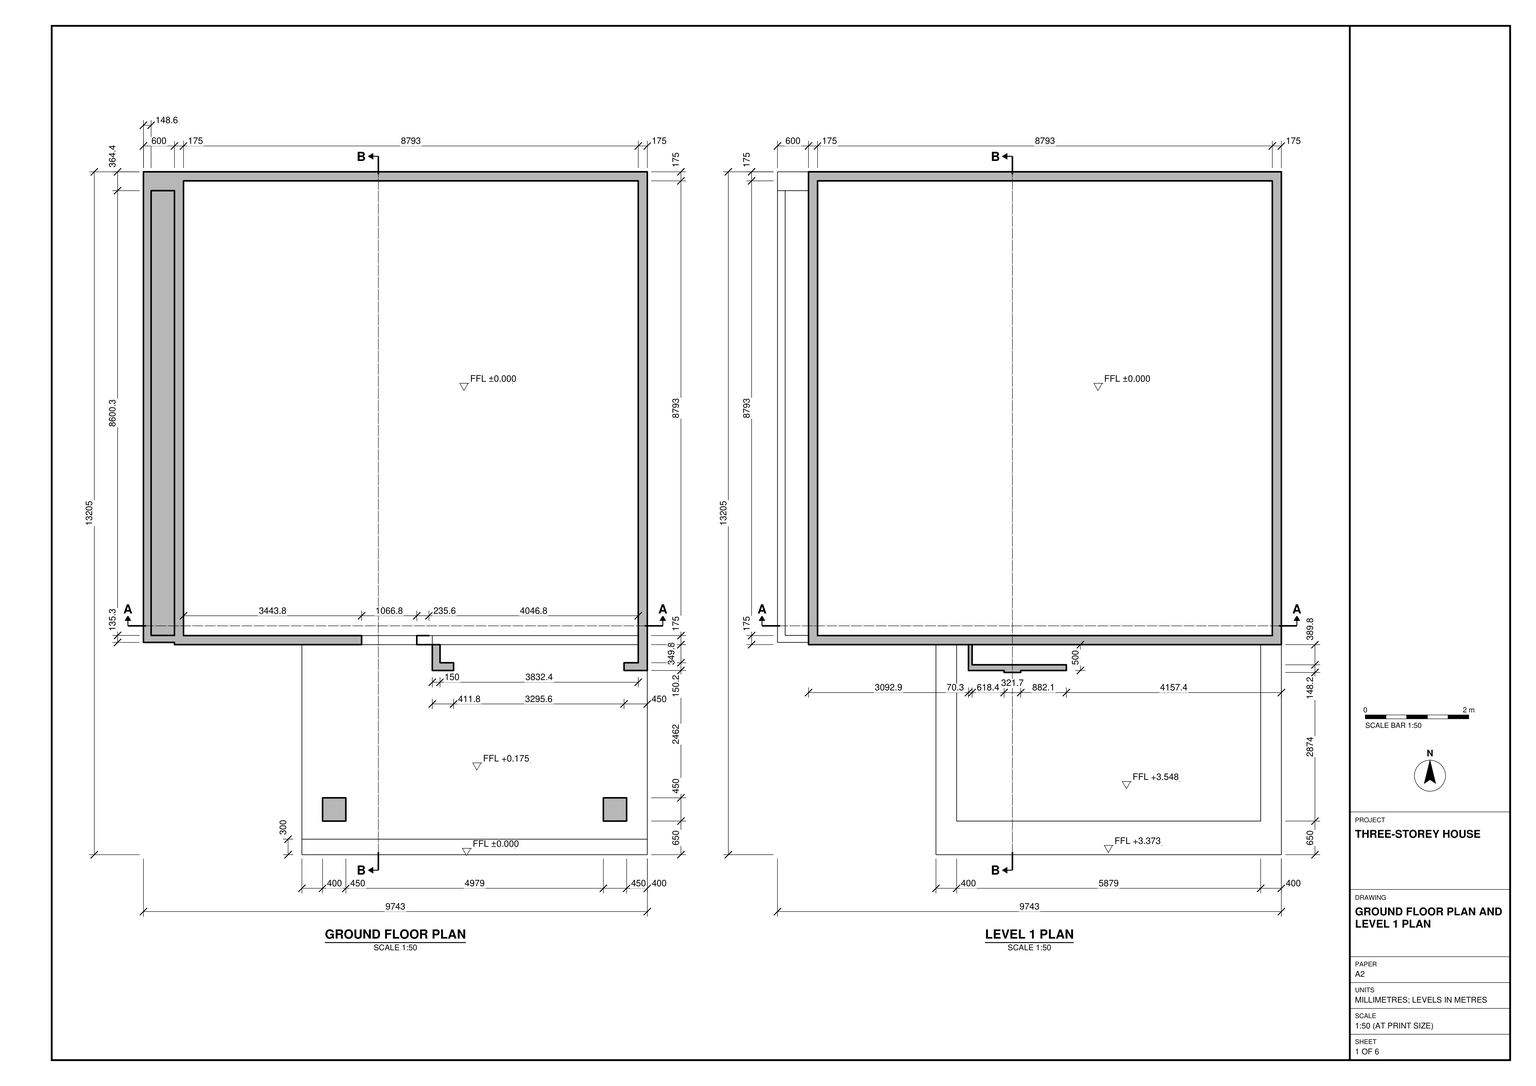
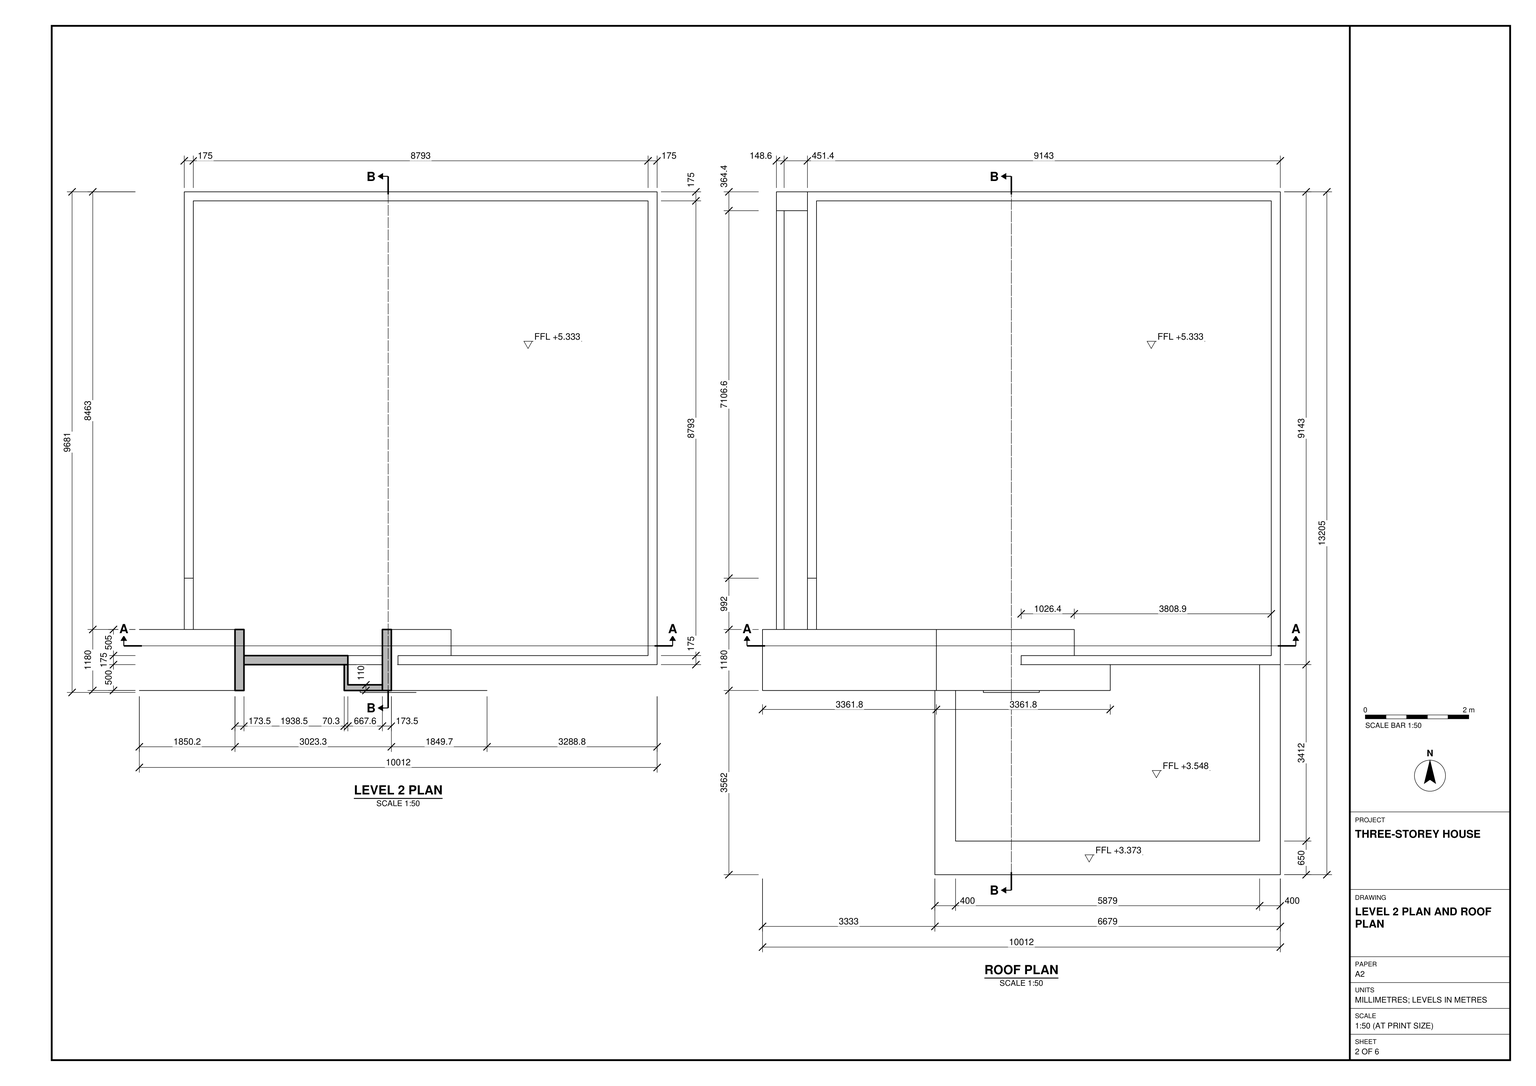
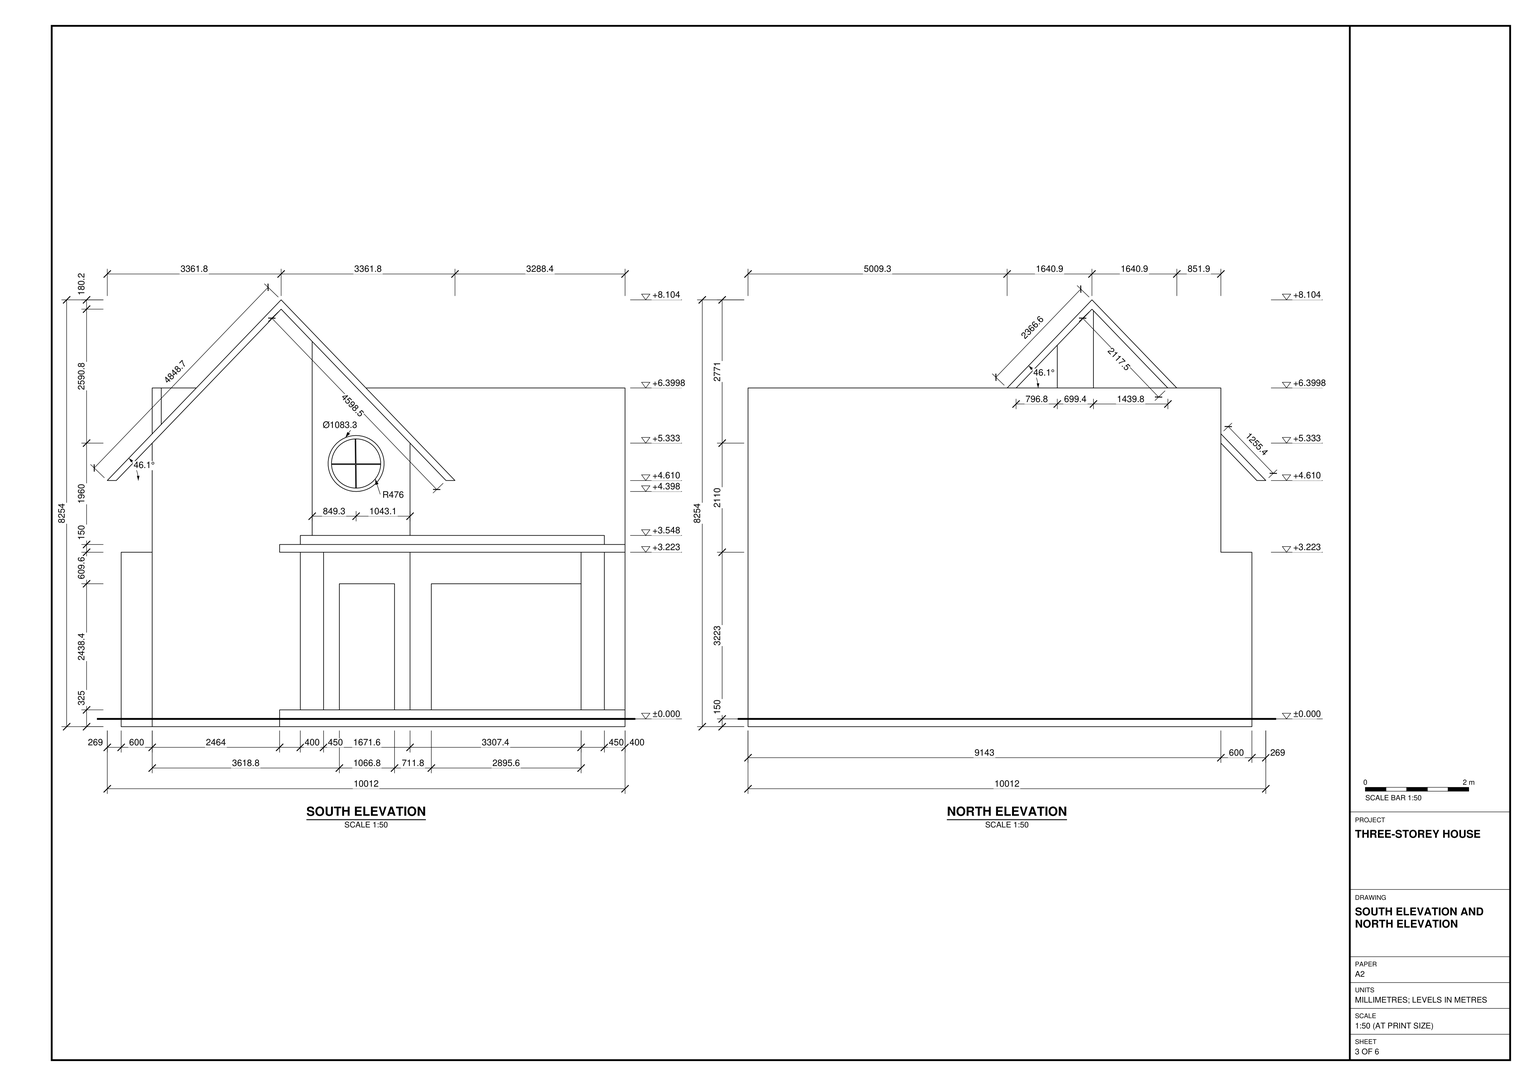
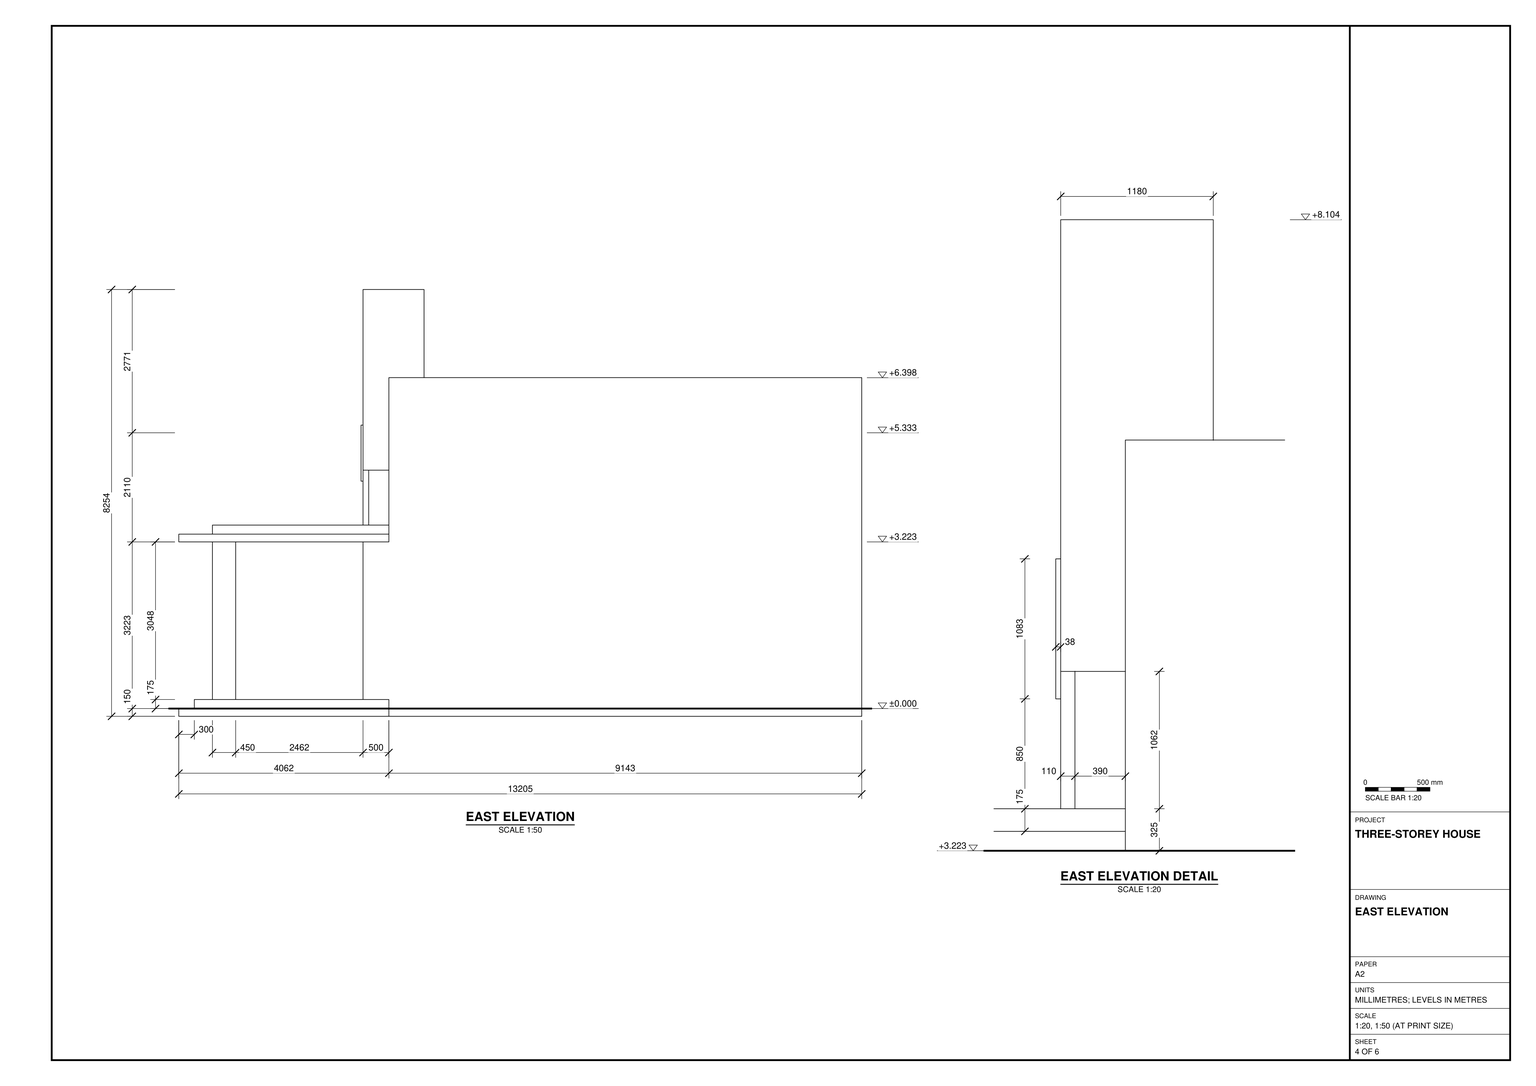
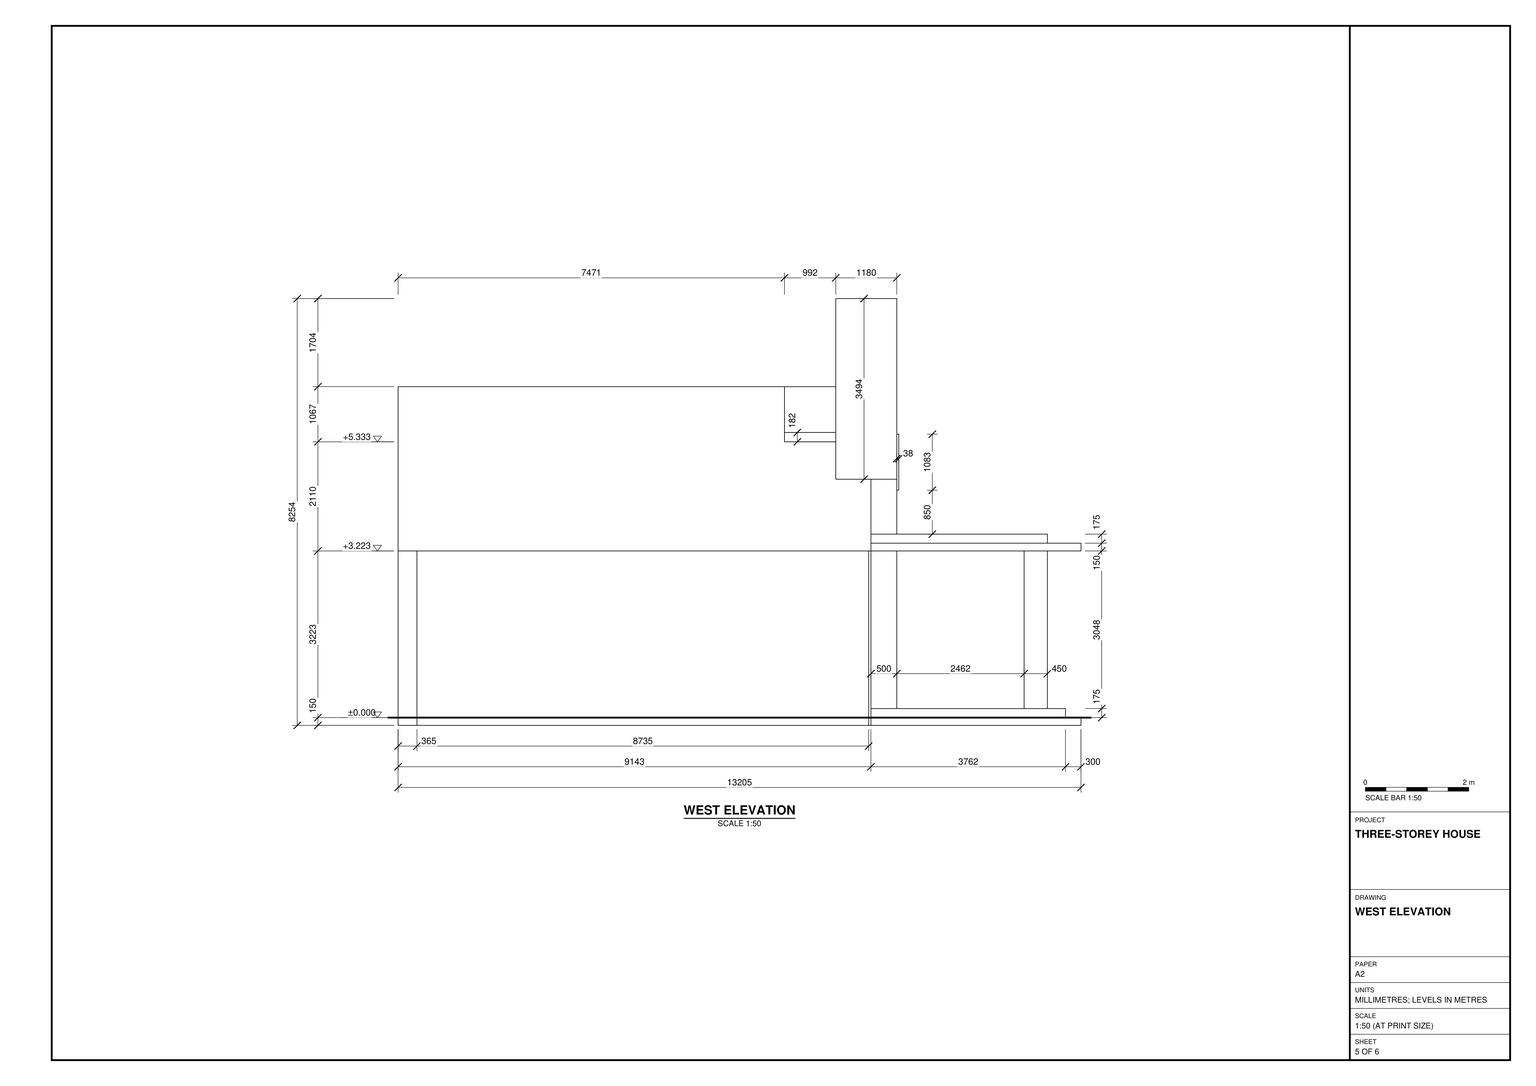
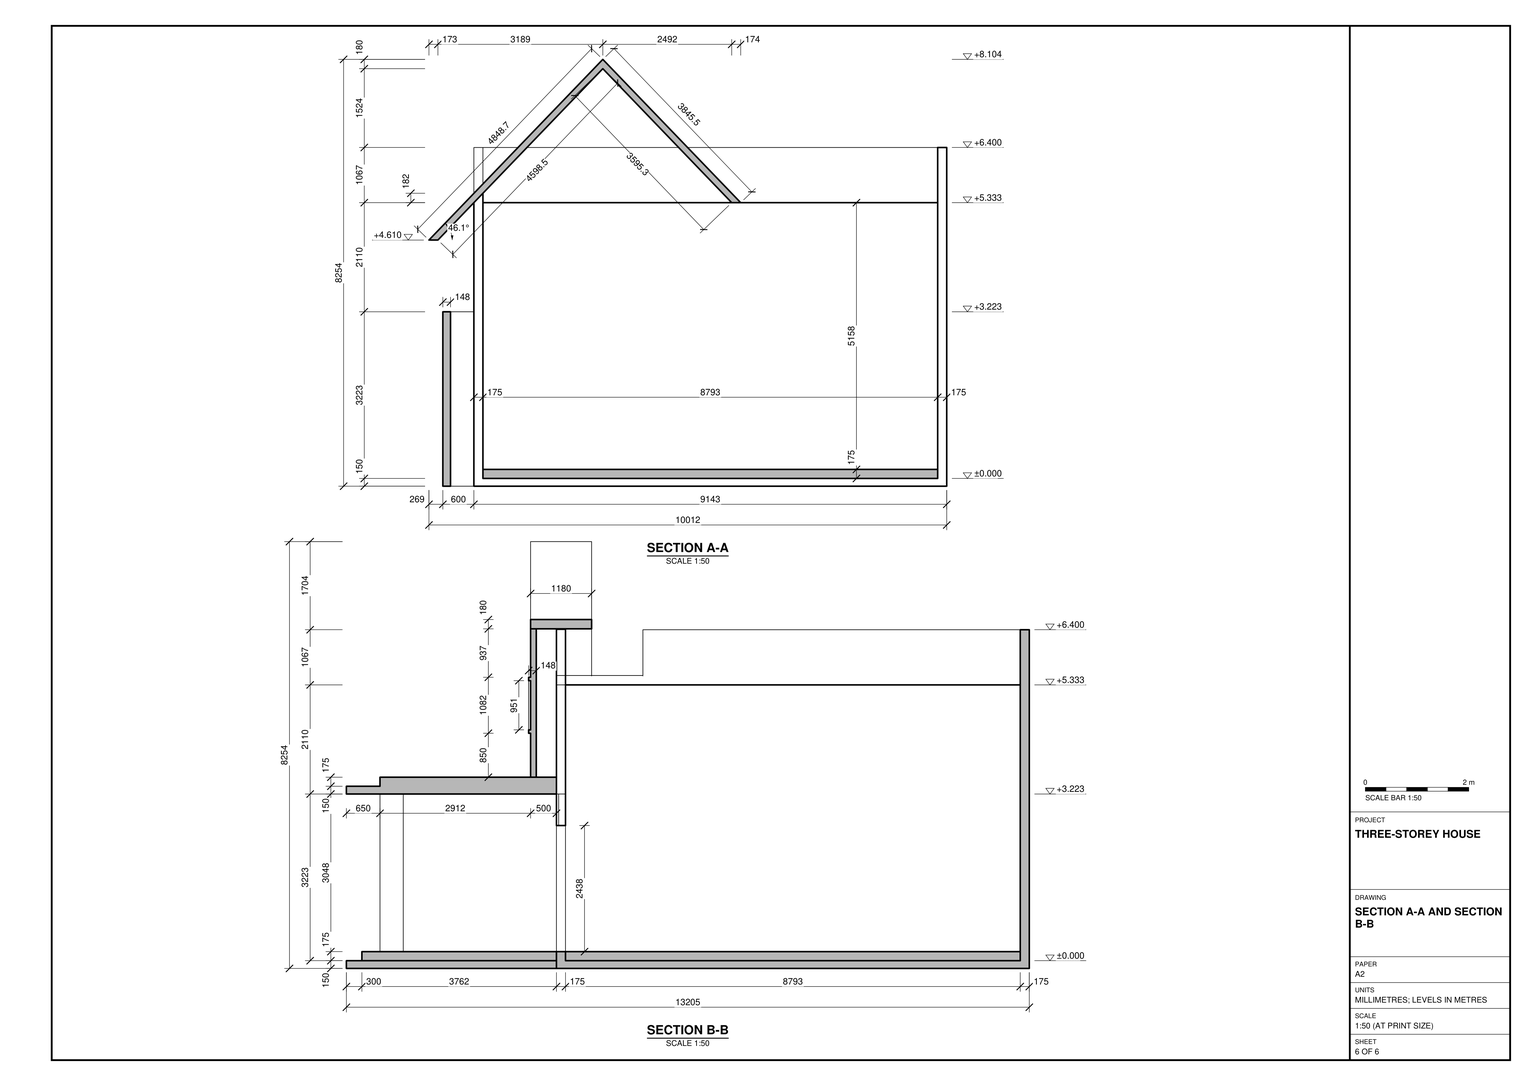
Build the three-storey house in SketchUp from task_files/diagram_01.pdf. Work in millimetres. Set the overall extents to 10012 mm east–west, 13205 mm north–south and 8254.1 mm vertically, including the projecting porch and roof edges. Use storey levels of 0 mm, +3223 mm and +5333 mm relative to the ground floor.

Lay out the square main block with 175 mm perimeter walls around an 8793 mm by 8793 mm interior. Follow the plans for the narrow strip along the west side and the offsets in the south wall. On the south side, model the raised porch platform, the flat cover and its square supports. Set the narrow entry opening and the wider rectangular bay behind the supports, using the plan to distinguish the wall returns from the posts. Above the porch, form the projecting gable with sloping edges that extend beyond its walls. Place the round window to the right of the ridge as seen from the south, and divide it with horizontal and vertical bars.

Keep walls, slabs, roof elements and any individual furniture or joinery pieces in separate groups or components; use components for repeated parts. Any decor or loose items shown may use suitable library components. Save one SketchUp model as output_files/three_storey_house_with_a_south_porch_and_gable.skp.

# SketchUp Ruby script. Lengths in millimetres.
U = 1.mm
M = Sketchup.active_model
def pt(a) = Geom::Point3d.new(a.map { |v| v * U })
def face(e, loops, mat)
  f = e.add_face(loops[0].map { |a| pt(a) })
  loops[1..].each { |l| e.add_face(l.map { |a| pt(a) }).erase! }
  f.material = f.back_material = mat if mat
  f
end
# faces: each face lists its corners as indices into pts; further lists are holes
def faces(e, pts, list, mat = nil) = list.each { |f| face(e, (f[0].is_a?(Array) ? f : [f]).map { |l| l.map { |i| pts[i] } }, mat) }
# xy, xz, yz: faces in a plane at the given z, y or x. An outline is a flat list of corners, or four numbers for a rectangle; further outlines are holes
def ring(l) = l.size == 4 ? [[l[0], l[1]], [l[2], l[1]], [l[2], l[3]], [l[0], l[3]]] : l.each_slice(2).to_a
def flat(e, list, mat, &to3) = list.each { |f| face(e, (f[0].is_a?(Array) ? f : [f]).map { |l| ring(l).map { |u, v| to3.(u, v) } }, mat) }
def xy(e, z, list, mat = nil) = flat(e, list, mat) { |x, y| [x, y, z] }
def xz(e, y, list, mat = nil) = flat(e, list, mat) { |x, z| [x, y, z] }
def yz(e, x, list, mat = nil) = flat(e, list, mat) { |y, z| [x, y, z] }
def lines(e, pts, list) = list.each { |a, b| e.add_line(pt(pts[a]), pt(pts[b])) }
# prism: a flat outline (further loops are holes) pulled along v
def prism(e, loops, v, mat = nil)
  f = face(e, loops, mat); d = Geom::Vector3d.new(v.map { |x| x * U })
  f.pushpull(f.normal.samedirection?(d) ? d.length : -d.length)
end
def box(e, o, s, mat = nil) = prism(e, [[o, [o[0] + s[0], o[1], o[2]], [o[0] + s[0], o[1] + s[1], o[2]], [o[0], o[1] + s[1], o[2]]]], [0, 0, s[2]], mat)
def at(x, y, z, deg = 0) = Geom::Transformation.translation(pt([x, y, z])) * Geom::Transformation.rotation(ORIGIN, Z_AXIS, deg.degrees)
def axes(o, x, y, z) = Geom::Transformation.new([*x, 0, *y, 0, *z, 0, *pt(o).to_a, 1])
def part(name) = M.definitions.add(name)
# library, detail: a bought-in or finely detailed component or shape, given as its bounding box
def library(name, o, s) = part(name).tap { |d| box(d.entities, o, s) }
def detail(e, o, s) = box(e.add_group.entities, o, s)
def put(e, d, t, mat = nil) = e.add_instance(d, t).tap { |i| i.material = mat if mat }
def group(e, t, mat = nil) = e.add_group.tap { |g| g.transformation = t; g.material = mat if mat }.entities
root = M.entities
xy(root,0,[[[869,4062,869,4105,269,4105,269,13205,10012,13205,10012,4062],[417.6,4240.3,869,12840.6]]])
xy(root,150,[[1044,4237,9837,13030]])
xy(root,325,[[5854.6,3562,6266.4,3712],[9562,3562,9562,3712,9837,3712,9837,4062,10012,4062,10012,3562],[5854.6,3712,6004.6,4062],[4487.8,4062,5554.6,4237],[5854.6,4062,9837,4237],
  [1044,4237,9837,13030]])
xy(root,2763.4,[[6266.4,3562,9562,3712],[4487.8,4062,5554.6,4237]])
xy(root,3373,[[5854.6,3562,10012,3562,10012,4062,9837,4062,9837,3712,5854.6,3712],[5854.6,3712,6004.6,4062],[269,4105,869,4105,869,4240.3,417.6,4240.3,417.6,12840.6,269,12840.6],[269,12840.6,869,13205]])
xy(root,3698,[[3962.2,3562,3962.2,4062,4032.4,4062,4032.4,3672.2,5854.6,3672.2,5854.6,3562]])
xy(root,4760.1,[[0,3562,173.5,4742],[6550.2,3562,6723.7,4237]])
xy(root,5483,[[1044,4237,5854.6,4237,5854.6,4742,6028.1,4742,6028.1,4237,9837,4237,9837,13030,1044,13030],[5854.6,4237,6028.1,4742]])
xy(root,6549.8,[[5001.7,4062,10012,4062,10012,13205,869,13205,869,5734,1044,5734,1044,13030,9837,13030,9837,4237,5001.7,4237]])
xz(root,3524,[[[4817.7,4547.6,4885.5,4552.6,4952.2,4566.1,5016.6,4587.9,5077.9,4617.5,5134.9,4654.7,5186.8,4698.6,5232.8,4748.7,5272.1,4804.2,5304.2,4864.2,5328.5,4927.7,5344.7,4993.8,5352.4,5061.4,5351.7,5129.4,5342.4,5196.8,5324.7,5262.5,5298.9,5325.4,5265.5,5384.7,5224.9,5439.2,5177.7,5488.3,5124.8,5531,5067,5566.8,5005.1,5595.1,4940.2,5615.3,4873.2,5627.3,4805.3,5630.8,4737.4,5625.8,4670.8,5612.3,4606.3,5590.5,4545.1,5560.8,4488.1,5523.7,4436.2,5479.8,4390.2,5429.7,4350.8,5374.2,4318.8,5314.2,4294.4,5250.7,4278.3,5184.6,4270.5,5117,4271.3,5049,4280.6,4981.6,4298.3,4915.9,4324,4853,4357.5,4793.7,4398.1,4739.2,4445.2,4690.1,4498.1,4647.3,4556,4611.6,4617.9,4583.3,4682.8,4563,4749.8,4551.1],[4816.9,4613.2,4757.2,4616.3,4698.4,4626.8,4641.3,4644.6,4587,4669.5,4536.1,4700.9,4489.6,4738.5,4448.2,4781.6,4412.5,4829.5,4383.1,4881.6,4360.5,4936.9,4345,4994.6,4336.8,5053.9,4336.1,5113.6,4342.9,5173,4357.1,5231.1,4378.5,5286.9,4406.7,5339.6,4441.3,5388.4,4481.7,5432.4,4527.3,5471,4577.4,5503.7,4631.2,5529.7,4687.8,5548.8,4746.4,5560.7,4806,5565.2,4865.7,5562.1,4924.6,5551.6,4981.6,5533.7,5036,5508.9,5086.8,5477.5,5133.3,5439.9,5174.7,5396.8,5210.4,5348.8,5239.8,5296.8,5262.5,5241.5,5278,5183.7,5286.2,5124.5,5286.9,5064.7,5280,5005.4,5265.8,4947.3,5244.5,4891.5,5216.3,4838.8,5181.7,4790,5141.3,4746,5095.7,4707.3,5045.6,4674.7,4991.8,4648.7,4935.1,4629.5,4876.5,4617.7]]])
xz(root,3562,[[5854.6,325,6266.4,325,6266.4,2763.4,9562,2763.4,9562,325,10012,325,10012,3373,5854.6,3373],[[3962.2,3698,5854.6,3698,5854.6,5483,4032.4,7376.8,3962.2,7449.9],[4817.7,4547.6,4749.8,4551.1,4682.8,4563,4617.9,4583.3,4556,4611.6,4498.1,4647.3,4445.2,4690.1,4398.1,4739.2,4357.5,4793.7,4324,4853,4298.3,4915.9,4280.6,4981.6,4271.3,5049,4270.5,5117,4278.3,5184.6,4294.4,5250.7,4318.8,5314.2,4350.8,5374.2,4390.2,5429.7,4436.2,5479.8,4488.1,5523.7,4545.1,5560.8,4606.3,5590.5,4670.8,5612.3,4737.4,5625.8,4805.3,5630.8,4873.2,5627.3,4940.2,5615.3,5005.1,5595.1,5067,5566.8,5124.8,5531,5177.7,5488.3,5224.9,5439.2,5265.5,5384.7,5298.9,5325.4,5324.7,5262.5,5342.4,5196.8,5351.7,5129.4,5352.4,5061.4,5344.7,4993.8,5328.5,4927.7,5304.2,4864.2,5272.1,4804.2,5232.8,4748.7,5186.8,4698.6,5134.9,4654.7,5077.9,4617.5,5016.6,4587.9,4952.2,4566.1,4885.5,4552.6]],[4816.9,4613.2,4876.5,4617.7,4935.1,4629.5,4991.8,4648.7,5045.6,4674.7,5095.7,4707.3,5141.3,4746,5181.7,4790,5216.3,4838.8,5244.5,4891.5,5265.8,4947.3,5280,5005.4,5286.9,5064.7,5286.6,5083.7,4811.5,5083.7,4806,5565.2,4792.1,5564.1,4797.6,5083.7,4336.4,5083.7,4336.6,5068.7,4336.8,5053.9,4345,4994.6,4360.5,4936.9,4383.1,4881.6,4412.5,4829.5,4448.2,4781.6,4489.6,4738.5,4536.1,4700.9,4587,4669.5,4641.3,4644.6,4698.4,4626.8,4757.2,4616.3,4803,4613.9],[0,4760.1,173.5,4760.1,3361.8,8073.8,3962.2,7449.9,4032.4,7376.8,5854.6,5483,6550.2,4760.1,6723.7,4760.1,3361.8,8254.1],[4336.4,5083.7,4797.6,5083.7,4792.1,5564.1,4746.4,5560.7,4687.8,5548.8,4631.2,5529.7,4577.4,5503.7,4527.3,5471,4481.7,5432.4,4441.3,5388.4,4406.7,5339.6,4378.5,5286.9,4357.1,5231.1,4342.9,5173,4336.1,5113.6],
  [4811.5,5083.7,5286.6,5083.7,5286.2,5124.5,5278,5183.7,5262.5,5241.5,5239.8,5296.8,5210.4,5348.8,5174.7,5396.8,5133.3,5439.9,5086.8,5477.5,5036,5508.9,4981.6,5533.7,4924.6,5551.6,4865.7,5562.1,4806,5565.2]])
xz(root,3672.2,[[4032.4,3698,4032.4,7376.8,5854.6,5483,5854.6,3698]])
xz(root,3712,[[6004.6,325,6004.6,3373,9837,3373,9837,325,9562,325,9562,2763.4,6266.4,2763.4,6266.4,325]])
xz(root,4062,[[[869,0,3333,0,3333,150,9837,150,9837,325,5854.6,325,5854.6,3373,10012,3373,10012,6549.8,4032.4,6549.8,4032.4,3698,3962.2,3698,3962.2,7449.9,3361.8,8073.8,1044,5664.9,869,5483],[4487.8,325,5554.6,2763.4]],[3333,0,10012,150],[9837,150,10012,325],[5854.6,325,6004.6,3097.9],[5854.6,3097.9,6004.6,3373],
  [3962.2,3698,4032.4,3698,4032.4,7376.8,3962.2,7449.9]])
xz(root,4105,[[269,0,869,3373]])
xz(root,4237,[[1044,150,3333,325],[3333,150,5790.4,325],[5790.4,150,9837,325],[1044,325,3333,5483],[3333,325,3333,5483,5790.4,5483,5790.4,325,5554.6,325,5554.6,2763.4,4487.8,2763.4,4487.8,325],
  [5790.4,3097.9,5790.4,5483,5854.6,5483,6550.2,4760.1,6723.7,4760.1,6028.1,5483,9837,5483,9837,3097.9],[6550.2,4760.1,5854.6,5483,6028.1,5483,6723.7,4760.1],[1044,5483,1044,5664.9,3333,8043.9,3333,5483],[3333,5483,3333,8043.9,3361.8,8073.8,3962.2,7449.9,4032.4,7376.8,4032.4,6549.8,4828.2,6549.8,5790.4,5549.8,5790.4,5483],[6028.1,5483,5001.7,6549.8,9837,6549.8,9837,5483],
  [5790.4,5483,5790.4,5549.8,5854.6,5483]])
xz(root,4240.3,[[417.6,0,869,3373]])
xz(root,4742,[[0,4760.1,3361.8,8254.1,6028.1,5483,5854.6,5483,5790.4,5549.8,4828.2,6549.8,4032.4,7376.8,3962.2,7449.9,3361.8,8073.8,3333,8043.9,1044,5664.9,869,5483,173.5,4760.1]])
xz(root,5734,[[869,5483,1044,5664.9,869,5664.9],[869,5664.9,1044,6549.8]])
xz(root,12840.6,[[417.6,0,869,3373]])
xz(root,13030,[[1044,150,9837,325],[1044,325,9837,5483],[1044,5483,9837,6549.8]])
xz(root,13205,[[269,0,269,3373,869,3373,869,6549.8,10012,6549.8,10012,0]])
yz(root,269,[[4105,0,12840.6,3373],[12840.6,0,13205,3373]])
yz(root,417.6,[[4240.3,0,12840.6,3373]])
yz(root,869,[[4062,0,4105,3373],[4240.3,0,4240.3,3373,4062,3373,4062,5483,5734,5483,5734,6549.8,13205,6549.8,13205,3373,12840.6,3373,12840.6,0]])
yz(root,1044,[[4237,150,13030,325],[4237,325,13030,5483],[4237,5483,13030,5483,13030,6549.8,5734,6549.8,5734,5664.9,4237,5664.9]])
yz(root,3962.2,[[3562,3698,4062,7449.9]])
yz(root,4032.4,[[3672.2,3698,4062,7376.8],[4062,6549.8,4237,7376.8]])
yz(root,4487.8,[[4062,325,4237,2763.4]])
yz(root,5554.6,[[4062,325,4237,2763.4]])
yz(root,5854.6,[[3562,325,4062,3373],[3562,3698,3672.2,5483]])
yz(root,6004.6,[[3712,325,4062,3373]])
yz(root,6266.4,[[3562,325,3712,2763.4]])
yz(root,9562,[[3562,325,3712,2763.4]])
yz(root,9837,[[4062,150,4237,325],[4237,150,13030,325],[3712,325,4237,3373],[4237,325,13030,5483],[4237,5483,13030,6549.8]])
yz(root,10012,[[4062,0,13205,0,13205,6549.8,4062,6549.8,4062,3373,3562,3373,3562,325,4062,325]])
p = [[4749.8,3562,4551.1],[4817.7,3562,4547.6],[4817.7,3524,4547.6],[4749.8,3524,4551.1],[4885.5,3562,4552.6],[4885.5,3524,4552.6],
  [4682.8,3562,4563],[4682.8,3524,4563],[4952.2,3562,4566.1],[4952.2,3524,4566.1],[4617.9,3562,4583.3],[4617.9,3524,4583.3],
  [5016.6,3562,4587.9],[5016.6,3524,4587.9],[4556,3562,4611.6],[4556,3524,4611.6],[5077.9,3562,4617.5],[5077.9,3524,4617.5],
  [4498.1,3562,4647.3],[4498.1,3524,4647.3],[4816.9,3562,4613.2],[4803,3562,4613.9],[4757.2,3562,4616.3],[4757.2,3524,4616.3],
  [4816.9,3524,4613.2],[4876.5,3562,4617.7],[4876.5,3524,4617.7],[4698.4,3562,4626.8],[4698.4,3524,4626.8],[5134.9,3562,4654.7],
  [5134.9,3524,4654.7],[4935.1,3562,4629.5],[4935.1,3524,4629.5],[4641.3,3562,4644.6],[4641.3,3524,4644.6],[4991.8,3562,4648.7],
  [4991.8,3524,4648.7],[4587,3562,4669.5],[4587,3524,4669.5],[4445.2,3562,4690.1],[4445.2,3524,4690.1],[5045.6,3562,4674.7],
  [5045.6,3524,4674.7],[5186.8,3562,4698.6],[5186.8,3524,4698.6],[4536.1,3562,4700.9],[4536.1,3524,4700.9],[5095.7,3562,4707.3],
  [5095.7,3524,4707.3],[4398.1,3562,4739.2],[4398.1,3524,4739.2],[5232.8,3562,4748.7],[5232.8,3524,4748.7],[4489.6,3562,4738.5],
  [4489.6,3524,4738.5],[5141.3,3562,4746],[5141.3,3524,4746],[4448.2,3562,4781.6],[4448.2,3524,4781.6],[4357.5,3562,4793.7],
  [4357.5,3524,4793.7],[5181.7,3562,4790],[5181.7,3524,4790],[5272.1,3562,4804.2],[5272.1,3524,4804.2],[0,3562,4760.1],
  [3361.8,3562,8254.1],[3361.8,4742,8254.1],[0,4742,4760.1],[173.5,3562,4760.1],[173.5,4742,4760.1],[869,4742,5483],
  [869,4062,5483],[1044,4062,5664.9],[3361.8,4062,8073.8],[3361.8,3562,8073.8],[6723.7,4237,4760.1],[6028.1,4237,5483],
  [6028.1,4742,5483],[6723.7,3562,4760.1],[6550.2,3562,4760.1],[5854.6,3562,5483],[5854.6,3672.2,5483],[5854.6,4237,5483],
  [6550.2,4237,4760.1],[4412.5,3562,4829.5],[4412.5,3524,4829.5],[5216.3,3562,4838.8],[5216.3,3524,4838.8],[4324,3562,4853],
  [4324,3524,4853],[5304.2,3562,4864.2],[5304.2,3524,4864.2],[4383.1,3562,4881.6],[4383.1,3524,4881.6],[5244.5,3562,4891.5],
  [5244.5,3524,4891.5],[4298.3,3562,4915.9],[4298.3,3524,4915.9],[5328.5,3562,4927.7],[5328.5,3524,4927.7],[4360.5,3562,4936.9],
  [4360.5,3524,4936.9],[5265.8,3562,4947.3],[5265.8,3524,4947.3],[4280.6,3562,4981.6],[4280.6,3524,4981.6],[5344.7,3562,4993.8],
  [5344.7,3524,4993.8],[4345,3562,4994.6],[4345,3524,4994.6],[5280,3562,5005.4],[5280,3524,5005.4],[4271.3,3562,5049],
  [4271.3,3524,5049],[5352.4,3562,5061.4],[5352.4,3524,5061.4],[4336.8,3562,5053.9],[4336.8,3524,5053.9],[5286.9,3562,5064.7],
  [5286.9,3524,5064.7],[4270.5,3562,5117],[4270.5,3524,5117],[4336.6,3562,5068.7],[4336.4,3562,5083.7],[4336.1,3562,5113.6],
  [4336.1,3524,5113.6],[5351.7,3562,5129.4],[5351.7,3524,5129.4],[5286.2,3562,5124.5],[5286.6,3562,5083.7],[5286.2,3524,5124.5],
  [4342.9,3562,5173],[4342.9,3524,5173],[4278.3,3562,5184.6],[4278.3,3524,5184.6],[5278,3562,5183.7],[5278,3524,5183.7],
  [5342.4,3562,5196.8],[5342.4,3524,5196.8],[4357.1,3562,5231.1],[4357.1,3524,5231.1],[5262.5,3562,5241.5],[5262.5,3524,5241.5],
  [4294.4,3562,5250.7],[4294.4,3524,5250.7],[5324.7,3562,5262.5],[5324.7,3524,5262.5],[4378.5,3562,5286.9],[4378.5,3524,5286.9],
  [5239.8,3562,5296.8],[5239.8,3524,5296.8],[4318.8,3562,5314.2],[4318.8,3524,5314.2],[5298.9,3562,5325.4],[5298.9,3524,5325.4],
  [4406.7,3562,5339.6],[4406.7,3524,5339.6],[5210.4,3562,5348.8],[5210.4,3524,5348.8],[4350.8,3562,5374.2],[4350.8,3524,5374.2],
  [5265.5,3562,5384.7],[5265.5,3524,5384.7],[4441.3,3562,5388.4],[4441.3,3524,5388.4],[5174.7,3562,5396.8],[5174.7,3524,5396.8],
  [4390.2,3562,5429.7],[4390.2,3524,5429.7],[5224.9,3562,5439.2],[5224.9,3524,5439.2],[4481.7,3562,5432.4],[4481.7,3524,5432.4],
  [5133.3,3562,5439.9],[5133.3,3524,5439.9],[4436.2,3562,5479.8],[4436.2,3524,5479.8],[4527.3,3562,5471],[4527.3,3524,5471],
  [5177.7,3562,5488.3],[5177.7,3524,5488.3],[5086.8,3562,5477.5],[5086.8,3524,5477.5],[4577.4,3562,5503.7],[4577.4,3524,5503.7],
  [5036,3562,5508.9],[5036,3524,5508.9],[4488.1,3562,5523.7],[4488.1,3524,5523.7],[4032.4,3672.2,7376.8],[4032.4,3562,7376.8],
  [4032.4,4062,7376.8],[4032.4,4237,7376.8],[4032.4,4742,7376.8],[4828.2,4742,6549.8],[4828.2,4237,6549.8],[5790.4,4237,5549.8],
  [1044,4237,5664.9],[1044,4742,5664.9],[5790.4,4742,5549.8],[5854.6,4742,5483],[869,5734,5483],[1044,5734,5664.9],
  [5124.8,3562,5531],[5124.8,3524,5531],[4631.2,3562,5529.7],[4631.2,3524,5529.7],[4981.6,3562,5533.7],[4981.6,3524,5533.7],
  [4545.1,3562,5560.8],[4545.1,3524,5560.8],[4687.8,3562,5548.8],[4687.8,3524,5548.8],[5067,3562,5566.8],[5067,3524,5566.8],
  [4924.6,3562,5551.6],[4924.6,3524,5551.6],[4746.4,3562,5560.7],[4746.4,3524,5560.7],[4865.7,3562,5562.1],[4865.7,3524,5562.1],
  [4792.1,3562,5564.1],[4806,3562,5565.2],[4806,3524,5565.2],[4606.3,3562,5590.5],[4606.3,3524,5590.5],[5005.1,3562,5595.1],
  [5005.1,3524,5595.1],[4670.8,3562,5612.3],[4670.8,3524,5612.3],[4940.2,3562,5615.3],[4940.2,3524,5615.3],[4737.4,3562,5625.8],
  [4737.4,3524,5625.8],[4873.2,3562,5627.3],[4873.2,3524,5627.3],[4805.3,3562,5630.8],[4805.3,3524,5630.8],[3333,4237,8043.9],
  [3361.8,4237,8073.8],[3333,4742,8043.9],[3962.2,3562,7449.9],[3962.2,4062,7449.9],[3962.2,4237,7449.9],[3962.2,4742,7449.9],
  [3361.8,4742,8073.8],[5790.4,4237,3097.9],[6004.6,4062,3097.9],[5854.6,4062,3698],[6014.7,4062,3698],[4797.6,3562,5083.7],
  [4797.6,3562,5082.7],[4803,3562,4612.2],[4811.5,3562,5068.7],[4811.7,3562,5068.7],[4336.4,3562,5068.7],[5286.6,3562,5068.7],
  [4797.6,3562,5068.7],[4797.7,3562,5068.5],[4797.9,3562,5054.3],[4798.1,3562,5040.1],[4798.2,3562,5025.9],[4798.4,3562,5011.7],
  [4798.6,3562,4997.5],[4798.7,3562,4983.3],[4798.9,3562,4969.1],[4799,3562,4954.9],[4799.2,3562,4940.7],[4799.4,3562,4926.4],
  [4799.5,3562,4912.2],[4799.7,3562,4898],[4799.9,3562,4883.8],[4800,3562,4869.6],[4800.2,3562,4855.4],[4800.3,3562,4841.2],
  [4800.5,3562,4827],[4800.7,3562,4812.8],[4800.8,3562,4798.6],[4801,3562,4784.4],[4801.2,3562,4770.2],[4801.3,3562,4756],
  [4801.5,3562,4741.8],[4801.7,3562,4727.6],[4801.8,3562,4713.4],[4802,3562,4699.2],[4802.1,3562,4685],[4802.3,3562,4670.8],
  [4802.5,3562,4656.6],[4802.6,3562,4642.3],[4802.8,3562,4628.1]]
faces(root,p,[[0,1,2,3],[1,4,5,2],[6,0,3,7],[4,8,9,5],[10,6,7,11],[8,12,13,9],[14,10,11,15],[12,16,17,13],
  [18,14,15,19],[20,21,22,23,24],[25,20,24,26],[22,27,28,23],[16,29,30,17],[31,25,26,32],[27,33,34,28],[35,31,32,36],
  [33,37,38,34],[39,18,19,40],[41,35,36,42],[29,43,44,30],[37,45,46,38],[47,41,42,48],[49,39,40,50],[43,51,52,44],
  [45,53,54,46],[55,47,48,56],[53,57,58,54],[59,49,50,60],[61,55,56,62],[51,63,64,52],[65,66,67,68],[69,70,71,72,73,74,75],
  [76,77,78,67,66,79],[80,81,82,83,84],[57,85,86,58],[87,61,62,88],[89,59,60,90],[63,91,92,64],[85,93,94,86],[95,87,88,96],
  [97,89,90,98],[91,99,100,92],[93,101,102,94],[103,95,96,104],[105,97,98,106],[99,107,108,100],[101,109,110,102],[111,103,104,112],
  [113,105,106,114],[107,115,116,108],[109,117,118,110],[119,111,112,120],[121,113,114,122],[117,123,124,125,126,118],[115,127,128,116],[129,130,119,120,131],
  [125,132,133,126],[134,121,122,135],[136,129,131,137],[127,138,139,128],[132,140,141,133],[142,136,137,143],[144,134,135,145],[138,146,147,139],
  [140,148,149,141],[150,142,143,151],[152,144,145,153],[146,154,155,147],[148,156,157,149],[158,150,151,159],[160,152,153,161],[154,162,163,155],
  [156,164,165,157],[166,158,159,167],[168,160,161,169],[162,170,171,163],[164,172,173,165],[174,166,167,175],[176,168,169,177],[172,178,179,173],
  [170,180,181,171],[182,174,175,183],[178,184,185,179],[186,182,183,187],[188,176,177,189],[190,82,81,191],[83,82,190,192,193,194,195,196,197],[73,198,199,71,72],
  [83,197,200,201],[202,71,199,203],[180,204,205,181],[184,206,207,185],[208,186,187,209],[210,188,189,211],[206,212,213,207],[204,214,215,205],
  [216,208,209,217],[212,218,219,213],[197,196,195,200],[220,216,217,221],[218,222,223,224,219],[225,210,211,226],[223,220,221,224],[214,227,228,215],
  [229,225,226,230],[227,231,232,228],[233,229,230,234],[231,235,236,232],[237,233,234,238],[235,237,238,236],[239,240,74,73,198],[239,198,199,241],
  [190,191,242,243,192],[193,244,243,192],[193,244,245,194],[75,74,243,242],[74,243,244,240],[244,240,246,245],[240,239,241,246]])
lines(root,p,[[247,248],[249,250],[251,252],[21,253],[254,255],[256,123],[255,20],[255,257],[123,258],[259,260],[260,261],[261,262],
  [262,263],[263,264],[264,265],[265,266],[266,267],[267,268],[268,269],[269,270],[270,271],[271,272],[272,273],[273,274],
  [274,275],[275,276],[276,277],[277,278],[278,279],[279,280],[280,281],[281,282],[282,283],[283,284],[284,285],[285,286],
  [286,287],[287,288],[288,289],[289,290],[290,21]])
g1 = group(root,at(3333,0,0))
xy(g1,0,[[0,0,6679,4062]])
xy(g1,150,[[0,0,6679,300],[0,300,6679,4062]])
xy(g1,325,[[[0,300,6679,4062],[5829,650,6279,1100],[400,650,850,1100]]])
xy(g1,3373,[[[0,0,6679,4062],[5829,650,6279,1100],[400,650,850,1100]],[400,650,850,1100],[5829,650,6279,1100]])
xy(g1,3523,[[0,0,6679,0,6679,4062,6279,4062,6279,650,400,650,400,4062,0,4062]])
xy(g1,3698,[[400,650,6279,4062]])
xz(g1,0,[[0,0,6679,150],[0,3373,6679,3523]])
xz(g1,300,[[0,150,6679,325]])
xz(g1,650,[[400,325,850,3373],[5829,325,6279,3373],[400,3523,6279,3698]])
xz(g1,1100,[[400,325,850,3373],[5829,325,6279,3373]])
xz(g1,4062,[[0,0,6679,150],[0,150,6679,325],[0,3373,0,3523,400,3523,400,3698,6279,3698,6279,3523,6679,3523,6679,3373]])
yz(g1,0,[[0,0,4062,150],[300,150,4062,325],[0,3373,4062,3523]])
yz(g1,400,[[650,325,1100,3373],[650,3523,4062,3698]])
yz(g1,850,[[650,325,1100,3373]])
yz(g1,5829,[[650,325,1100,3373]])
yz(g1,6279,[[650,325,1100,3373],[650,3523,4062,3698]])
yz(g1,6679,[[0,0,4062,150],[300,150,4062,325],[0,3373,4062,3523]])
